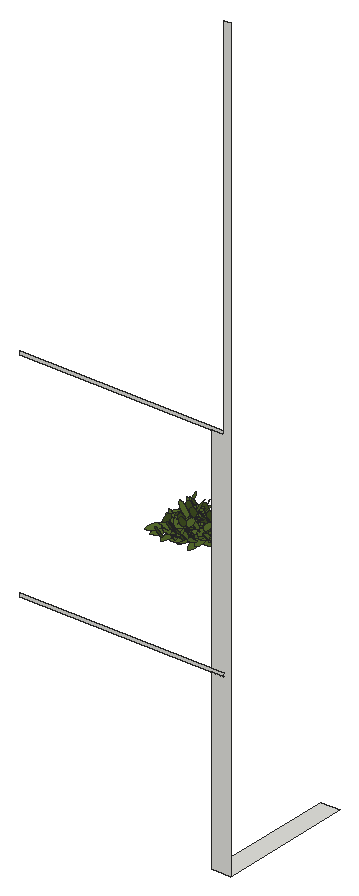
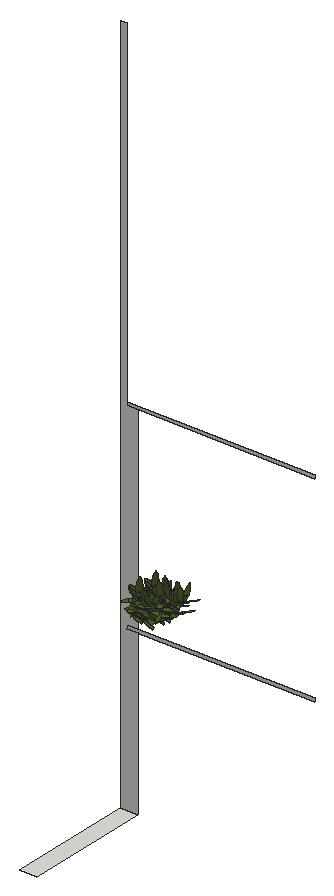
# SketchUp Ruby script. Lengths in inches.
U = 1.inch
M = Sketchup.active_model
def pt(a) = Geom::Point3d.new(a.map { |v| v * U })
def face(e, loops, mat)
  f = e.add_face(loops[0].map { |a| pt(a) })
  loops[1..].each { |l| e.add_face(l.map { |a| pt(a) }).erase! }
  f.material = f.back_material = mat if mat
  f
end
# faces: each face lists its corners as indices into pts; further lists are holes
def faces(e, pts, list, mat = nil) = list.each { |f| face(e, (f[0].is_a?(Array) ? f : [f]).map { |l| l.map { |i| pts[i] } }, mat) }
# xy, xz, yz: faces in a plane at the given z, y or x. An outline is a flat list of corners, or four numbers for a rectangle; further outlines are holes
def ring(l) = l.size == 4 ? [[l[0], l[1]], [l[2], l[1]], [l[2], l[3]], [l[0], l[3]]] : l.each_slice(2).to_a
def flat(e, list, mat, &to3) = list.each { |f| face(e, (f[0].is_a?(Array) ? f : [f]).map { |l| ring(l).map { |u, v| to3.(u, v) } }, mat) }
def xy(e, z, list, mat = nil) = flat(e, list, mat) { |x, y| [x, y, z] }
def xz(e, y, list, mat = nil) = flat(e, list, mat) { |x, z| [x, y, z] }
def yz(e, x, list, mat = nil) = flat(e, list, mat) { |y, z| [x, y, z] }
def lines(e, pts, list) = list.each { |a, b| e.add_line(pt(pts[a]), pt(pts[b])) }
# prism: a flat outline (further loops are holes) pulled along v
def prism(e, loops, v, mat = nil)
  f = face(e, loops, mat); d = Geom::Vector3d.new(v.map { |x| x * U })
  f.pushpull(f.normal.samedirection?(d) ? d.length : -d.length)
end
def box(e, o, s, mat = nil) = prism(e, [[o, [o[0] + s[0], o[1], o[2]], [o[0] + s[0], o[1] + s[1], o[2]], [o[0], o[1] + s[1], o[2]]]], [0, 0, s[2]], mat)
def at(x, y, z, deg = 0) = Geom::Transformation.translation(pt([x, y, z])) * Geom::Transformation.rotation(ORIGIN, Z_AXIS, deg.degrees)
def axes(o, x, y, z) = Geom::Transformation.new([*x, 0, *y, 0, *z, 0, *pt(o).to_a, 1])
def part(name) = M.definitions.add(name)
# library, detail: a bought-in or finely detailed component or shape, given as its bounding box
def library(name, o, s) = part(name).tap { |d| box(d.entities, o, s) }
def detail(e, o, s) = box(e.add_group.entities, o, s)
def put(e, d, t, mat = nil) = e.add_instance(d, t).tap { |i| i.material = mat if mat }
def group(e, t, mat = nil) = e.add_group.tap { |g| g.transformation = t; g.material = mat if mat }.entities
root = M.entities
M.materials.add("[Asphalt_New]").color = [85, 106, 44]
M.materials.add("white").color = [255, 255, 255]
c1 = part("Component\#59")
xy(c1.entities,0,[[5.79,0,4.75,0.06,3.73,0.22,2.73,0.5,1.77,0.88,0.86,1.37,0,1.95,0.83,2.59,1.74,3.13,2.7,3.56,3.7,3.87,4.74,4.05,5.79,4.12,6.84,4.05,7.87,3.87,8.88,3.56,9.84,3.13,10.74,2.59,11.57,1.95,10.72,1.37,9.8,0.88,8.84,0.5,7.84,0.22,6.82,0.06]],"[Asphalt_New]")
c2 = part("Leaf cluster")
put(c2.entities,c1,axes([10.37,9.23,1.73],[-0.67725,-0.67301,0.29729],[0.61625,-0.73963,-0.27052],[0.40195,0,0.91566]),"[Asphalt_New]")
put(c2.entities,c1,at(0,5.84,1.2),"[Asphalt_New]")
put(c2.entities,c1,axes([11.625,9.72,1.52],[-0.61694,-0.11161,0.77906],[-0.02647,-0.98639,-0.16227],[0.78657,-0.12073,0.60559]),"[Asphalt_New]")
put(c2.entities,c1,axes([13.35,8.05,1.98],[-0.1211,0.99122,-0.05316],[-0.90762,-0.13226,-0.39842],[-0.40195,0,0.91566]),"[Asphalt_New]")
xy(root,41,[[147.625,9,149.5625,23.51]])
xz(root,9,[[147.625,41,149.5625,41,149.5625,122.4375,148.875,122.4375,148.875,82.88,147.625,82.88,147.625,60.22,148.875,60.22,148.875,59.82,147.625,59.82],[127.1875,59.82,148.875,60.22],[127.1875,82.88,148.875,83.28]])
put(root,c2,axes([140.5,14.72,67.45],[-0.12016,0.09321,0],[-0.09321,-0.12016,0],[0,0,0.17792]),"white")
put(root,c2,axes([140.54,13.99,68.22],[-0.12016,0.09321,0],[-0.09321,-0.12016,0],[0,0,0.17792]),"white")
put(root,c1,axes([138.03,14.47,68.25],[0.14768,-0.03627,0],[0.03627,0.14768,0],[0,0,0.17792]),"[Asphalt_New]")
put(root,c1,axes([138.16,14.6875,67.625],[0.15184,-0.00221,-0.00946],[-0.00119,0.13948,-0.07089],[0.0083,0.06056,0.16292]),"[Asphalt_New]")
put(root,c1,axes([138.68,13.21,67.77],[0.01154,-0.09464,0.13861],[0.14952,-0.01265,-0.02887],[0.02521,0.11836,0.10775]),"[Asphalt_New]")
put(root,c1,axes([138.2,13.97,68.4],[0.15184,-0.00221,-0.00946],[-0.00119,0.13948,-0.07089],[0.0083,0.06056,0.16292]),"[Asphalt_New]")
put(root,c1,axes([139.68,14.6,68.34],[-0.12443,-0.07482,0.0529],[0.06418,-0.13158,-0.04813],[0.05936,-0.01458,0.16292]),"[Asphalt_New]")
put(root,c1,axes([139.49,17.37,68.34],[-0.09806,-0.10708,0.0529],[0.09891,-0.10794,-0.04813],[0.06106,0.00288,0.16292]),"[Asphalt_New]")
put(root,c2,axes([138.97,14.86,67.61],[0.12994,0.079,0],[-0.079,0.12994,0],[0,0,0.17792]),"white")
put(root,c1,axes([139.41,12.8,67.71],[0.00875,0.15182,0],[-0.15182,0.00875,0],[0,0,0.17792]),"[Asphalt_New]")
put(root,c1,axes([139.68,17.45,68.3],[-0.09292,-0.02137,0.13861],[0.00305,-0.15002,-0.02887],[0.12035,-0.0127,0.10775]),"[Asphalt_New]")
put(root,c2,axes([139.86,13.41,67.26],[0.07604,0.1317,0],[-0.1317,0.07604,0],[0,0,0.17792]),"white")
put(root,c1,axes([138.4,17.08,67.78],[0.09625,-0.10871,0.0529],[0.11768,0.08708,-0.04813],[0.00352,0.06102,0.16292]),"[Asphalt_New]")
put(root,c1,axes([139.89,14.62,68.31],[-0.09516,0.0059,0.13861],[-0.03969,-0.14471,-0.02887],[0.11178,-0.04636,0.10775]),"[Asphalt_New]")
put(root,c2,axes([140.89,15.67,67.45],[-0.12303,0.08939,0],[-0.08939,-0.12303,0],[0,0,0.17792]),"white")
put(root,c2,axes([137.58,16.11,67.4],[0.09591,-0.11801,0],[0.11801,0.09591,0],[0,0,0.17792]),"white")
put(root,c1,axes([138.92,14.6,67.77],[0.01154,-0.09464,0.13861],[0.14952,-0.01265,-0.02887],[0.02521,0.11836,0.10775]),"[Asphalt_New]")
put(root,c2,axes([141.01,14.73,68.12],[-0.10136,0.11337,0],[-0.11337,-0.10136,0],[0,0,0.17792]),"white")
put(root,c2,axes([140.95,14.95,68.22],[-0.12303,0.08939,0],[-0.08939,-0.12303,0],[0,0,0.17792]),"white")
put(root,c2,axes([138.61,17.33,67.98],[-0.06975,-0.13513,0],[0.13513,-0.06975,0],[0,0,0.17792]),"white")
put(root,c2,axes([140.04,14.07,67.26],[0.07604,0.1317,0],[-0.1317,0.07604,0],[0,0,0.17792]),"white")
put(root,c1,axes([140.24,16.6,68.37],[-0.15155,-0.00971,-0.00946],[0.01213,-0.13895,-0.07089],[-0.00352,-0.06102,0.16292]),"[Asphalt_New]")
put(root,c1,axes([138.48,15.28,68.96],[0.14768,-0.03627,0],[0.03627,0.14768,0],[0,0,0.17792]),"[Asphalt_New]")
put(root,c1,axes([138.54,15.57,67.625],[0.15183,0.00256,-0.00946],[-0.00557,0.13937,-0.07089],[0.00639,0.06079,0.16292]),"[Asphalt_New]")
put(root,c1,axes([139.68,12.39,67.92],[0.00875,0.15182,0],[-0.15182,0.00875,0],[0,0,0.17792]),"[Asphalt_New]")
put(root,c1,axes([139.625,14.76,68.39],[0.01807,0.15078,-0.00946],[-0.13884,0.01339,-0.07089],[-0.05936,0.01458,0.16292]),"[Asphalt_New]")
put(root,c2,axes([137.77,16.78,67.4],[0.09591,-0.11801,0],[0.11801,0.09591,0],[0,0,0.17792]),"white")
put(root,c1,axes([138.61,14.85,68.4],[0.15183,0.00256,-0.00946],[-0.00557,0.13937,-0.07089],[0.00639,0.06079,0.16292]),"[Asphalt_New]")
put(root,c2,axes([137.9,16.39,68.2],[0.1271,-0.08349,0],[0.08349,0.1271,0],[0,0,0.17792]),"white")
put(root,c2,axes([141.2,16.75,67.57],[-0.10136,0.11337,0],[-0.11337,-0.10136,0],[0,0,0.17792]),"white")
put(root,c2,axes([141.22,15.64,68.83],[-0.10136,0.11337,0],[-0.11337,-0.10136,0],[0,0,0.17792]),"white")
put(root,c1,axes([140.14,15.41,69.06],[-0.12443,-0.07482,0.0529],[0.06418,-0.13158,-0.04813],[0.05936,-0.01458,0.16292]),"[Asphalt_New]")
put(root,c2,axes([138.8125,18.24,68.69],[-0.06975,-0.13513,0],[0.13513,-0.06975,0],[0,0,0.17792]),"white")
put(root,c1,axes([139.19,14.19,67.98],[0.01154,-0.09464,0.13861],[0.14952,-0.01265,-0.02887],[0.02521,0.11836,0.10775]),"[Asphalt_New]")
put(root,c2,axes([140.28,15.32,67.26],[0.07604,0.1317,0],[-0.1317,0.07604,0],[0,0,0.17792]),"white")
put(root,c2,axes([139.6875,16.75,67.81],[-0.12334,-0.08896,0],[0.08896,-0.12334,0],[0,0,0.17792]),"white")
put(root,c1,axes([139.93,15.38,68.95],[0.00875,0.15182,0],[-0.15182,0.00875,0],[0,0,0.17792]),"[Asphalt_New]")
put(root,c2,axes([141.33,17.03,67.47],[-0.12016,0.09321,0],[-0.09321,-0.12016,0],[0,0,0.17792]),"white")
put(root,c1,axes([140.55,14.24,67.85],[-0.15155,-0.00971,-0.00946],[0.01213,-0.13895,-0.07089],[-0.00352,-0.06102,0.16292]),"[Asphalt_New]")
put(root,c1,axes([140.34,15.4375,69.02],[-0.09516,0.0059,0.13861],[-0.03969,-0.14471,-0.02887],[0.11178,-0.04636,0.10775]),"[Asphalt_New]")
put(root,c1,axes([138.78,16.35,67.7],[0.14768,-0.03627,0],[0.03627,0.14768,0],[0,0,0.17792]),"[Asphalt_New]")
put(root,c1,axes([140.59,17.13,68.37],[-0.15155,-0.00971,-0.00946],[0.01213,-0.13895,-0.07089],[-0.00352,-0.06102,0.16292]),"[Asphalt_New]")
put(root,c2,axes([141.41,13.92,68.35],[-0.06499,0.13748,0],[-0.13748,-0.06499,0],[0,0,0.17792]),"white")
put(root,c1,axes([138.98,14.4,67.8],[0.09625,-0.10871,0.0529],[0.11768,0.08708,-0.04813],[0.00352,0.06102,0.16292]),"[Asphalt_New]")
put(root,c2,axes([138.21,14.03,67.67],[0.1271,-0.08349,0],[0.08349,0.1271,0],[0,0,0.17792]),"white")
put(root,c1,axes([139.4375,17.18,69],[0.01154,-0.09464,0.13861],[0.14952,-0.01265,-0.02887],[0.02521,0.11836,0.10775]),"[Asphalt_New]")
put(root,c1,axes([140.43,16.48,67.79],[-0.12443,-0.07482,0.0529],[0.06418,-0.13158,-0.04813],[0.05936,-0.01458,0.16292]),"[Asphalt_New]")
put(root,c1,axes([140.08,14.3125,68.39],[0.01807,0.15078,-0.00946],[-0.13884,0.01339,-0.07089],[-0.05936,0.01458,0.16292]),"[Asphalt_New]")
put(root,c1,axes([139.51,15.73,67.4375],[0.01842,-0.15074,-0.00946],[0.13802,0.02011,-0.07089],[0.06112,0,0.16292]),"[Asphalt_New]")
put(root,c2,axes([139.96,16.34,68.02],[-0.12334,-0.08896,0],[0.08896,-0.12334,0],[0,0,0.17792]),"white")
put(root,c1,axes([140.64,16.5,67.76],[-0.09516,0.0059,0.13861],[-0.03969,-0.14471,-0.02887],[0.11178,-0.04636,0.10775]),"[Asphalt_New]")
put(root,c1,axes([139.26,13.99,68.02],[0.09625,-0.10871,0.0529],[0.11768,0.08708,-0.04813],[0.00352,0.06102,0.16292]),"[Asphalt_New]")
put(root,c1,axes([139.7,16.39,67.4375],[0.01842,-0.15074,-0.00946],[0.13802,0.02011,-0.07089],[0.06112,0,0.16292]),"[Asphalt_New]")
put(root,c2,axes([139.84,17.09,68.21],[-0.10525,-0.10976,0],[0.10976,-0.10525,0],[0,0,0.17792]),"white")
put(root,c1,axes([140.45,14.56,68.23],[0.00875,0.15182,0],[-0.15182,0.00875,0],[0,0,0.17792]),"[Asphalt_New]")
put(root,c2,axes([141.87,13.48,68.35],[-0.06499,0.13748,0],[-0.13748,-0.06499,0],[0,0,0.17792]),"white")
put(root,c2,axes([141.9,16.92,68.34],[-0.10136,0.11337,0],[-0.11337,-0.10136,0],[0,0,0.17792]),"white")
put(root,c2,axes([140.89,13.39,67.05],[0.07604,0.1317,0],[-0.1317,0.07604,0],[0,0,0.17792]),"white")
put(root,c1,axes([139.5,16.98,69.04],[0.09625,-0.10871,0.0529],[0.11768,0.08708,-0.04813],[0.00352,0.06102,0.16292]),"[Asphalt_New]")
put(root,c2,axes([138.62,16.09,67.18],[0.09591,-0.11801,0],[0.11801,0.09591,0],[0,0,0.17792]),"white")
put(root,c2,axes([141.96,16.75,67.47],[-0.12016,0.09321,0],[-0.09321,-0.12016,0],[0,0,0.17792]),"white")
put(root,c1,axes([139.78,15.48,67.36],[0.09382,0.01697,0.13861],[0.00402,0.15,-0.02887],[-0.11961,0.01836,0.10775]),"[Asphalt_New]")
put(root,c1,axes([139.9375,17.64,67.4375],[0.01842,-0.15074,-0.00946],[0.13802,0.02011,-0.07089],[0.06112,0,0.16292]),"[Asphalt_New]")
put(root,c1,axes([139.97,16.35,68.29],[0.01154,-0.09464,0.13861],[0.14952,-0.01265,-0.02887],[0.02521,0.11836,0.10775]),"[Asphalt_New]")
put(root,c1,axes([140.53,15.125,69.1],[0.01807,0.15078,-0.00946],[-0.13884,0.01339,-0.07089],[-0.05936,0.01458,0.16292]),"[Asphalt_New]")
put(root,c1,axes([139.97,15.55,67.39],[0.10299,0.10235,0.0529],[-0.09371,0.11248,-0.04813],[-0.06112,0,0.16292]),"[Asphalt_New]")
put(root,c1,axes([139.5,16.3125,68.47],[0.14768,-0.03627,0],[0.03627,0.14768,0],[0,0,0.17792]),"[Asphalt_New]")
put(root,c2,axes([141.16,13.93,67.26],[0.07604,0.1317,0],[-0.1317,0.07604,0],[0,0,0.17792]),"white")
put(root,c1,axes([139.62,16.72,67.65],[0.15184,-0.00221,-0.00946],[-0.00119,0.13948,-0.07089],[0.0083,0.06056,0.16292]),"[Asphalt_New]")
put(root,c1,axes([139.96,16.14,67.36],[0.09382,0.01697,0.13861],[0.00402,0.15,-0.02887],[-0.11961,0.01836,0.10775]),"[Asphalt_New]")
put(root,c1,axes([140.81,15.08,68.23],[0.00875,0.15182,0],[-0.15182,0.00875,0],[0,0,0.17792]),"[Asphalt_New]")
put(root,c1,axes([140.15,16.21,67.39],[0.10299,0.10235,0.0529],[-0.09371,0.11248,-0.04813],[-0.06112,0,0.16292]),"[Asphalt_New]")
put(root,c1,axes([141.16,16.4375,68.57],[-0.12443,-0.07482,0.0529],[0.06418,-0.13158,-0.04813],[0.05936,-0.01458,0.16292]),"[Asphalt_New]")
put(root,c2,axes([138.88,16.64,67.4],[0.09591,-0.11801,0],[0.11801,0.09591,0],[0,0,0.17792]),"white")
put(root,c2,axes([140.3,16.65,68.21],[-0.10525,-0.10976,0],[0.10976,-0.10525,0],[0,0,0.17792]),"white")
put(root,c2,axes([142.32,14.29,69.06],[-0.06499,0.13748,0],[-0.13748,-0.06499,0],[0,0,0.17792]),"white")
put(root,c1,axes([140.28,13.99,67.77],[0.01154,-0.09464,0.13861],[0.14952,-0.01265,-0.02887],[0.02521,0.11836,0.10775]),"[Asphalt_New]")
put(root,c1,axes([141.54,16.07,67.3],[-0.15207,0,0],[0,-0.15207,0],[0,0,0.17792]),"[Asphalt_New]")
put(root,c1,axes([140.32,16.88,68.29],[0.01154,-0.09464,0.13861],[0.14952,-0.01265,-0.02887],[0.02521,0.11836,0.10775]),"[Asphalt_New]")
put(root,c2,axes([140.73,18.51,68.33],[-0.12334,-0.08896,0],[0.08896,-0.12334,0],[0,0,0.17792]),"white")
put(root,c1,axes([141.36,16.46,68.53],[-0.09516,0.0059,0.13861],[-0.03969,-0.14471,-0.02887],[0.11178,-0.04636,0.10775]),"[Asphalt_New]")
put(root,c1,axes([140.03,16.16,68.33],[0.09625,-0.10871,0.0529],[0.11768,0.08708,-0.04813],[0.00352,0.06102,0.16292]),"[Asphalt_New]")
put(root,c1,axes([141.73,16.73,67.3],[-0.15207,0,0],[0,-0.15207,0],[0,0,0.17792]),"[Asphalt_New]")
put(root,c1,axes([140.55,15.71,67.22],[0.01842,-0.15074,-0.00946],[0.13802,0.02011,-0.07089],[0.06112,0,0.16292]),"[Asphalt_New]")
put(root,c2,axes([142.62,15.36,67.8],[-0.06499,0.13748,0],[-0.13748,-0.06499,0],[0,0,0.17792]),"white")
put(root,c2,axes([141.68,15.16,67.26],[0.07604,0.1317,0],[-0.1317,0.07604,0],[0,0,0.17792]),"white")
put(root,c2,axes([140.75,17.46,68.92],[-0.10525,-0.10976,0],[0.10976,-0.10525,0],[0,0,0.17792]),"white")
put(root,c1,axes([140.38,16.6875,68.33],[0.09625,-0.10871,0.0529],[0.11768,0.08708,-0.04813],[0.00352,0.06102,0.16292]),"[Asphalt_New]")
put(root,c1,axes([140.82,16.25,67.4375],[0.01842,-0.15074,-0.00946],[0.13802,0.02011,-0.07089],[0.06112,0,0.16292]),"[Asphalt_New]")
put(root,c2,axes([141.05,18.53,67.66],[-0.10525,-0.10976,0],[0.10976,-0.10525,0],[0,0,0.17792]),"white")
put(root,c1,axes([140.8125,15.45,67.14],[0.09382,0.01697,0.13861],[0.00402,0.15,-0.02887],[-0.11961,0.01836,0.10775]),"[Asphalt_New]")
put(root,c1,axes([141.55,16.16,68.61],[0.01807,0.15078,-0.00946],[-0.13884,0.01339,-0.07089],[-0.05936,0.01458,0.16292]),"[Asphalt_New]")
put(root,c1,axes([141,15.52,67.18],[0.10299,0.10235,0.0529],[-0.09371,0.11248,-0.04813],[-0.06112,0,0.16292]),"[Asphalt_New]")
put(root,c1,axes([141.08,16,67.36],[0.09382,0.01697,0.13861],[0.00402,0.15,-0.02887],[-0.11961,0.01836,0.10775]),"[Asphalt_New]")
put(root,c1,axes([141.27,16.07,67.39],[0.10299,0.10235,0.0529],[-0.09371,0.11248,-0.04813],[-0.06112,0,0.16292]),"[Asphalt_New]")
put(root,c2,axes([143.34,15.32,68.57],[-0.06499,0.13748,0],[-0.13748,-0.06499,0],[0,0,0.17792]),"white")
put(root,c1,axes([142.58,16.04,67.09],[-0.15207,0,0],[0,-0.15207,0],[0,0,0.17792]),"[Asphalt_New]")
put(root,c1,axes([141.34,17.48,67.4375],[0.01842,-0.15074,-0.00946],[0.13802,0.02011,-0.07089],[0.06112,0,0.16292]),"[Asphalt_New]")
put(root,c1,axes([142.84,16.59,67.3],[-0.15207,0,0],[0,-0.15207,0],[0,0,0.17792]),"[Asphalt_New]")
put(root,c2,axes([141.77,18.49,68.4375],[-0.10525,-0.10976,0],[0.10976,-0.10525,0],[0,0,0.17792]),"white")
